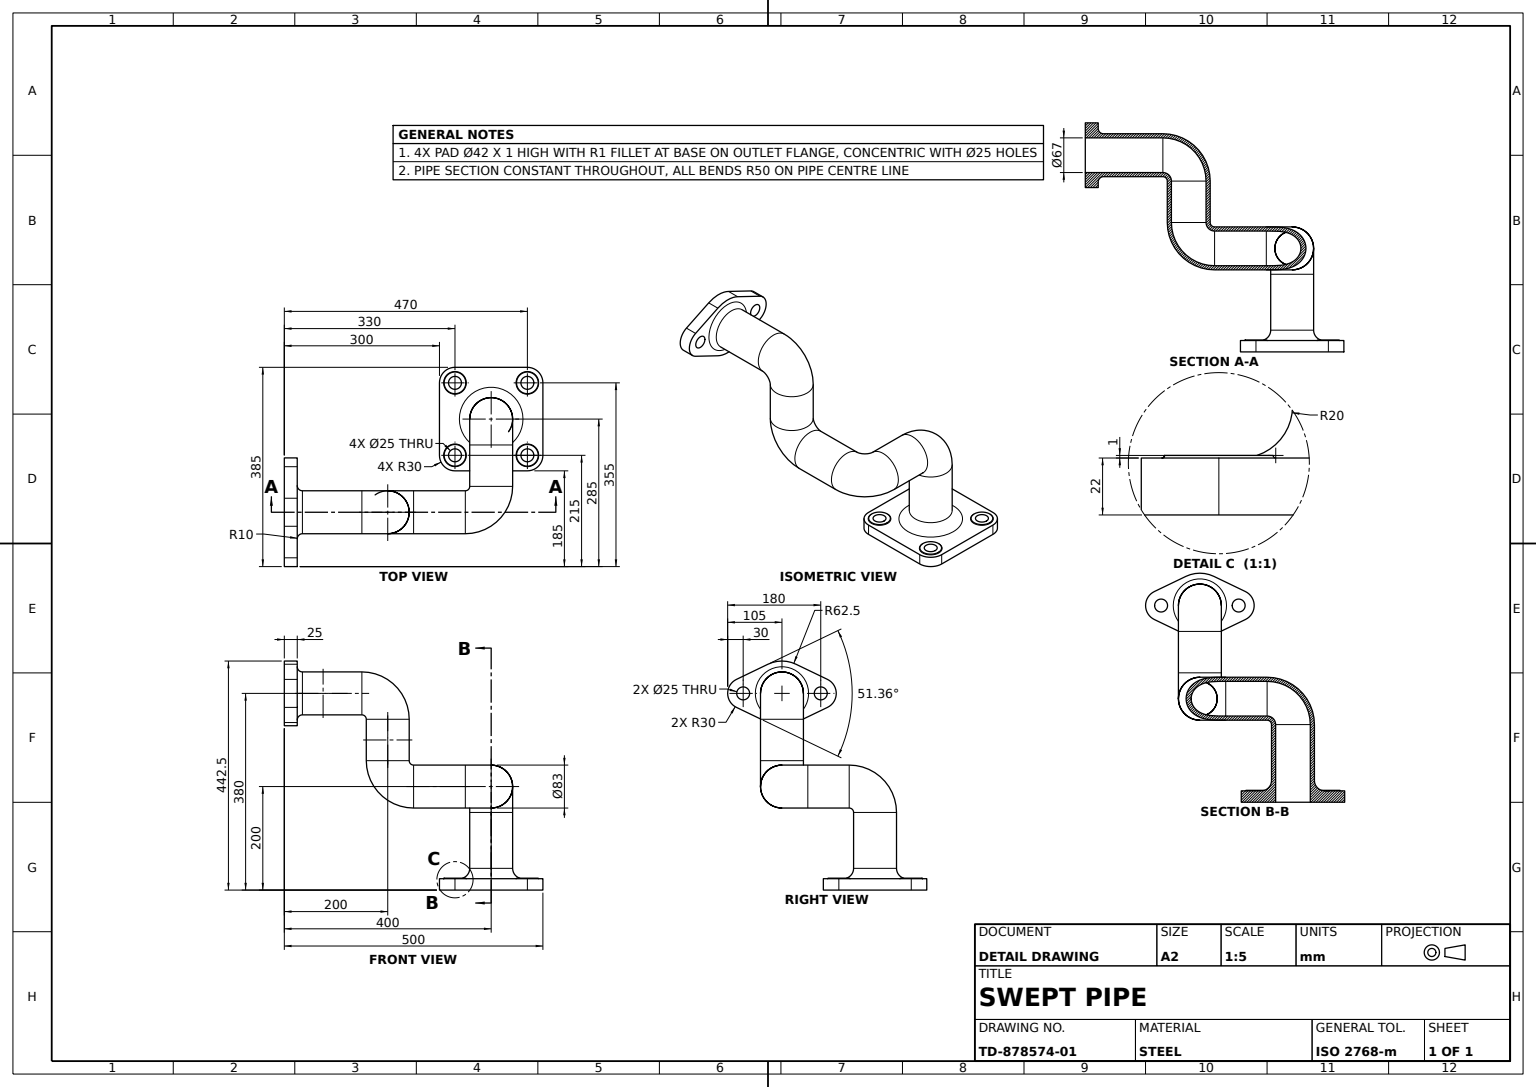
solid
v1 (70,23,49)
v2 (70,23,91)
e1 v1 v2 CIRCLE(AX(P(70,23,70),D(0,1,0),D(0,0,-1)),21)
v3 (70,22,48)
e2 v3 v1 CIRCLE(AX(P(70,23,48),D(-1,0,0),D(0,0,1)),1)
v4 (70,22,92)
e3 v4 v3 CIRCLE(AX(P(70,22,70),D(0,-1,0),D(0,0,-1)),22)
e4 v4 v2 CIRCLE(AX(P(70,23,92),D(1,0,0),D(0,0,-1)),1)
face TORUS(AX(P(70,23,70),D(0,-1,0),D(0,0,-1)),22,1) rev [-e1 -e2 -e3 e4]
v5 (100,22,-70)
v6 (100,0,-70)
e5 v5 v6 LINE
v7 (100,22,70)
e6 v5 v7 LINE
v8 (100,0,70)
e7 v7 v8 LINE
e8 v6 v8 LINE
face PLANE(AX(P(100,22,0),D(1,0,0),D(0,0,-1))) [-e5 e6 e7 -e8]
v9 (50,200,-33.5)
v10 (50,166.5,0)
e9 v9 v10 CIRCLE(AX(P(50,200,0),D(-1,0,0),D(0,-1,0)),33.5)
v11 (50,200,33.5)
e10 v10 v11 CIRCLE(AX(P(50,200,0),D(-1,0,0),D(0,-1,0)),33.5)
v12 (130,200,33.5)
e11 v11 v12 LINE
v13 (130,200,-33.5)
e12 v13 v12 CIRCLE(AX(P(130,200,0),D(-1,0,0),D(0,0,-1)),33.5)
e13 v9 v13 LINE
face CYL(AX(P(50,200,0),D(1,0,0),D(0,0,-1)),33.5) rev [e9 e10 e11 -e12 -e13]
v14 (130,200,-41.5)
v15 (130,200,41.5)
e14 v14 v15 CIRCLE(AX(P(130,200,0),D(-1,0,0),D(0,0,-1)),41.5)
v16 (221.5,200,50)
e15 v14 v16 CIRCLE(AX(P(130,200,50),D(0,-1,0),D(0,0,-1)),91.5)
v17 (138.5,200,50)
e16 v16 v17 CIRCLE(AX(P(180,200,50),D(0,0,-1),D(-1,0,0)),41.5)
e17 v15 v17 CIRCLE(AX(P(130,200,50),D(0,-1,0),D(0,0,-1)),8.5)
face TORUS(AX(P(130,200,50),D(0,-1,0),D(0,0,-1)),50,41.5) [-e14 e15 e16 -e17]
v18 (33.5,150,0)
v19 (0,150,33.5)
e18 v18 v19 CIRCLE(AX(P(0,150,0),D(0,-1,0),D(0,0,1)),33.5)
v20 (0,150,-33.5)
e19 v20 v18 CIRCLE(AX(P(0,150,0),D(0,-1,0),D(0,0,1)),33.5)
v21 (0,0,-33.5)
e20 v21 v20 LINE
v22 (0,0,33.5)
e21 v21 v22 CIRCLE(AX(P(0,0,0),D(0,-1,0),D(0,0,-1)),33.5)
e22 v22 v19 LINE
face CYL(AX(P(0,0,0),D(0,1,0),D(0,0,1)),33.5) rev [-e18 -e19 -e20 e21 e22]
v23 (221.5,380,250)
v24 (221.5,380,365)
e23 v23 v24 LINE
v25 (138.5,380,365)
e24 v24 v25 CIRCLE(AX(P(180,380,365),D(0,0,-1),D(1,0,0)),41.5)
v26 (138.5,380,250)
e25 v26 v25 LINE
v27 (180,338.5,250)
e26 v27 v26 CIRCLE(AX(P(180,380,250),D(0,0,-1),D(0,1,0)),41.5)
e27 v23 v27 CIRCLE(AX(P(180,380,250),D(0,0,-1),D(0,1,0)),41.5)
face CYL(AX(P(180,380,250),D(0,0,1),D(1,0,0)),41.5) [e23 e24 -e25 -e26 -e27]
v28 (213.5,330,200)
v29 (180,330,233.5)
e28 v28 v29 CIRCLE(AX(P(180,330,200),D(0,-1,0),D(-1,0,0)),33.5)
v30 (180,346.5,250)
e29 v29 v30 CIRCLE(AX(P(180,330,250),D(1,0,0),D(0,0,-1)),16.5)
v31 (213.5,380,250)
e30 v31 v30 CIRCLE(AX(P(180,380,250),D(0,0,-1),D(0,1,0)),33.5)
v32 (180,413.5,250)
e31 v32 v31 CIRCLE(AX(P(180,380,250),D(0,0,-1),D(0,1,0)),33.5)
v33 (180,330,166.5)
e32 v33 v32 CIRCLE(AX(P(180,330,250),D(1,0,0),D(0,0,-1)),83.5)
e33 v33 v28 CIRCLE(AX(P(180,330,200),D(0,-1,0),D(-1,0,0)),33.5)
face TORUS(AX(P(180,330,250),D(1,0,0),D(0,0,-1)),50,33.5) rev [e28 e29 -e30 -e31 -e32 e33]
v34 (-41.5,150,0)
v35 (50,241.5,0)
e34 v34 v35 CIRCLE(AX(P(50,150,0),D(0,0,-1),D(-1,0,0)),91.5)
v36 (0,150,41.5)
e35 v36 v34 CIRCLE(AX(P(0,150,0),D(0,-1,0),D(0,0,1)),41.5)
v37 (41.5,150,0)
e36 v37 v36 CIRCLE(AX(P(0,150,0),D(0,-1,0),D(0,0,1)),41.5)
v38 (50,158.5,0)
e37 v37 v38 CIRCLE(AX(P(50,150,0),D(0,0,-1),D(-1,0,0)),8.5)
v39 (50,200,41.5)
e38 v38 v39 CIRCLE(AX(P(50,200,0),D(-1,0,0),D(0,-1,0)),41.5)
e39 v39 v35 CIRCLE(AX(P(50,200,0),D(-1,0,0),D(0,-1,0)),41.5)
face TORUS(AX(P(50,150,0),D(0,0,-1),D(-1,0,0)),50,41.5) [-e34 -e35 -e36 e37 e38 e39]
v40 (92,407.037012,400)
v41 (92,352.962988,400)
e40 v40 v41 CIRCLE(AX(P(105,380,400),D(0,0,1),D(1,0,0)),30)
v42 (92,407.037012,375)
e41 v42 v40 LINE
v43 (92,352.962988,375)
e42 v42 v43 CIRCLE(AX(P(105,380,375),D(0,0,1),D(1,0,0)),30)
e43 v43 v41 LINE
face CYL(AX(P(105,380,375),D(0,0,1),D(1,0,0)),30) [-e40 -e41 e42 e43]
v44 (-70,0,82.5)
v45 (-70,0,57.5)
e44 v44 v45 CIRCLE(AX(P(-70,0,70),D(0,-1,0),D(0,0,-1)),12.5)
v46 (-70,23,57.5)
e45 v46 v45 LINE
v47 (-70,23,82.5)
e46 v46 v47 CIRCLE(AX(P(-70,23,70),D(0,1,0),D(1,0,0)),12.5)
e47 v47 v44 LINE
face CYL(AX(P(-70,22,70),D(0,-1,0),D(0,0,-1)),12.5) rev [e44 -e45 e46 e47]
v48 (146.5,380,400)
v49 (213.5,380,400)
e48 v48 v49 CIRCLE(AX(P(180,380,400),D(0,0,-1),D(-1,0,0)),33.5)
v50 (146.5,380,250)
e49 v50 v48 LINE
e50 v50 v32 CIRCLE(AX(P(180,380,250),D(0,0,-1),D(0,1,0)),33.5)
e51 v31 v49 LINE
face CYL(AX(P(180,380,250),D(0,0,1),D(1,0,0)),33.5) rev [-e48 -e49 e50 e31 e51]
v51 (70,23,-57.5)
v52 (70,0,-57.5)
e52 v51 v52 LINE
v53 (70,0,-82.5)
e53 v52 v53 CIRCLE(AX(P(70,0,-70),D(0,-1,0),D(0,0,-1)),12.5)
v54 (70,23,-82.5)
e54 v54 v53 LINE
e55 v54 v51 CIRCLE(AX(P(70,23,-70),D(0,1,0),D(-1,0,0)),12.5)
face CYL(AX(P(70,22,-70),D(0,-1,0),D(0,0,-1)),12.5) rev [e52 e53 -e54 e55]
e56 v47 v46 CIRCLE(AX(P(-70,23,70),D(0,1,0),D(1,0,0)),12.5)
v55 (-70,23,91)
v56 (-70,23,49)
e57 v55 v56 CIRCLE(AX(P(-70,23,70),D(0,1,0),D(1,0,0)),21)
e58 v56 v55 CIRCLE(AX(P(-70,23,70),D(0,1,0),D(1,0,0)),21)
face PLANE(AX(P(-70,23,70),D(0,1,0),D(1,0,0))) [-e46 -e56] [e57 e58]
v57 (268,407.037012,375)
v58 (268,407.037012,400)
e59 v57 v58 LINE
v59 (285,380,400)
e60 v59 v58 CIRCLE(AX(P(255,380,400),D(0,0,1),D(1,0,0)),30)
v60 (285,380,375)
e61 v60 v59 LINE
e62 v60 v57 CIRCLE(AX(P(255,380,375),D(0,0,1),D(1,0,0)),30)
face CYL(AX(P(255,380,375),D(0,0,1),D(1,0,0)),30) [e59 -e60 -e61 e62]
v61 (-70,23,-57.5)
v62 (-70,23,-82.5)
e63 v61 v62 CIRCLE(AX(P(-70,23,-70),D(0,1,0),D(0,0,1)),12.5)
v63 (-70,0,-82.5)
e64 v62 v63 LINE
v64 (-70,0,-57.5)
e65 v63 v64 CIRCLE(AX(P(-70,0,-70),D(0,-1,0),D(0,0,-1)),12.5)
e66 v61 v64 LINE
face CYL(AX(P(-70,22,-70),D(0,-1,0),D(0,0,-1)),12.5) rev [e63 e64 e65 -e66]
v65 (221.5,200,150)
v66 (180,158.5,150)
e67 v65 v66 CIRCLE(AX(P(180,200,150),D(0,0,-1),D(1,0,0)),41.5)
v67 (180,241.5,150)
e68 v67 v65 CIRCLE(AX(P(180,200,150),D(0,0,-1),D(1,0,0)),41.5)
v68 (180,250,158.5)
e69 v67 v68 CIRCLE(AX(P(180,250,150),D(-1,0,0),D(0,0,1)),8.5)
v69 (221.5,250,200)
e70 v68 v69 CIRCLE(AX(P(180,250,200),D(0,-1,0),D(0,0,-1)),41.5)
v70 (180,250,241.5)
e71 v69 v70 CIRCLE(AX(P(180,250,200),D(0,-1,0),D(0,0,-1)),41.5)
e72 v66 v70 CIRCLE(AX(P(180,250,150),D(-1,0,0),D(0,0,1)),91.5)
face TORUS(AX(P(180,250,150),D(-1,0,0),D(0,0,1)),50,41.5) [-e67 -e68 e69 e70 e71 -e72]
v71 (70,22,-48)
v72 (70,23,-49)
e73 v71 v72 CIRCLE(AX(P(70,23,-48),D(1,0,0),D(0,0,-1)),1)
v73 (70,22,-92)
e74 v73 v71 CIRCLE(AX(P(70,22,-70),D(0,-1,0),D(0,0,-1)),22)
v74 (70,23,-91)
e75 v73 v74 CIRCLE(AX(P(70,23,-92),D(-1,0,0),D(0,0,1)),1)
e76 v72 v74 CIRCLE(AX(P(70,23,-70),D(0,1,0),D(-1,0,0)),21)
face TORUS(AX(P(70,23,-70),D(0,-1,0),D(0,0,-1)),22,1) rev [-e73 -e74 e75 -e76]
e77 v49 v48 CIRCLE(AX(P(180,380,400),D(0,0,-1),D(-1,0,0)),33.5)
e78 v30 v50 CIRCLE(AX(P(180,380,250),D(0,0,-1),D(0,1,0)),33.5)
face CYL(AX(P(180,380,250),D(0,0,1),D(1,0,0)),33.5) rev [e49 -e77 -e51 e30 e78]
v75 (117.5,380,400)
v76 (92.5,380,400)
e79 v75 v76 CIRCLE(AX(P(105,380,400),D(0,0,1),D(1,0,0)),12.5)
v77 (92.5,380,375)
e80 v77 v76 LINE
v78 (117.5,380,375)
e81 v78 v77 CIRCLE(AX(P(105,380,375),D(0,0,1),D(1,0,0)),12.5)
e82 v78 v75 LINE
face CYL(AX(P(105,380,375),D(0,0,1),D(1,0,0)),12.5) rev [e79 -e80 -e81 e82]
e83 v15 v14 CIRCLE(AX(P(130,200,0),D(-1,0,0),D(0,0,-1)),41.5)
e84 v17 v16 CIRCLE(AX(P(180,200,50),D(0,0,-1),D(-1,0,0)),41.5)
face TORUS(AX(P(130,200,50),D(0,-1,0),D(0,0,-1)),50,41.5) [-e83 e17 e84 -e15]
v79 (138.5,200,150)
e85 v17 v79 LINE
e86 v79 v67 CIRCLE(AX(P(180,200,150),D(0,0,-1),D(1,0,0)),41.5)
e87 v16 v65 LINE
face CYL(AX(P(180,200,50),D(0,0,1),D(1,0,0)),41.5) [-e84 e85 e86 e68 -e87]
v80 (146.5,250,200)
v81 (146.5,330,200)
e88 v80 v81 LINE
v82 (180,250,166.5)
e89 v80 v82 CIRCLE(AX(P(180,250,200),D(0,-1,0),D(0,0,-1)),33.5)
v83 (213.5,250,200)
e90 v82 v83 CIRCLE(AX(P(180,250,200),D(0,-1,0),D(0,0,-1)),33.5)
e91 v83 v28 LINE
e92 v81 v33 CIRCLE(AX(P(180,330,200),D(0,-1,0),D(-1,0,0)),33.5)
face CYL(AX(P(180,250,200),D(0,1,0),D(-1,0,0)),33.5) rev [-e88 e89 e90 e91 -e33 -e92]
v84 (-70,23,-91)
v85 (-70,23,-49)
e93 v84 v85 CIRCLE(AX(P(-70,23,-70),D(0,1,0),D(0,0,1)),21)
e94 v85 v84 CIRCLE(AX(P(-70,23,-70),D(0,1,0),D(0,0,1)),21)
e95 v62 v61 CIRCLE(AX(P(-70,23,-70),D(0,1,0),D(0,0,1)),12.5)
face PLANE(AX(P(-70,23,-70),D(0,1,0),D(0,0,1))) [e93 e94] [-e63 -e95]
v86 (213.5,200,150)
v87 (180,166.5,150)
e96 v86 v87 CIRCLE(AX(P(180,200,150),D(0,0,-1),D(1,0,0)),33.5)
v88 (180,250,233.5)
e97 v87 v88 CIRCLE(AX(P(180,250,150),D(-1,0,0),D(0,0,1)),83.5)
e98 v83 v88 CIRCLE(AX(P(180,250,200),D(0,-1,0),D(0,0,-1)),33.5)
v89 (180,233.5,150)
e99 v89 v82 CIRCLE(AX(P(180,250,150),D(-1,0,0),D(0,0,1)),16.5)
e100 v89 v86 CIRCLE(AX(P(180,200,150),D(0,0,-1),D(1,0,0)),33.5)
face TORUS(AX(P(180,250,150),D(-1,0,0),D(0,0,1)),50,33.5) rev [e96 e97 -e98 -e90 -e99 e100]
v90 (-70,22,-48)
e101 v90 v85 CIRCLE(AX(P(-70,23,-48),D(1,0,0),D(0,0,-1)),1)
v91 (-70,22,-92)
e102 v91 v84 CIRCLE(AX(P(-70,23,-92),D(-1,0,0),D(0,0,1)),1)
e103 v90 v91 CIRCLE(AX(P(-70,22,-70),D(0,-1,0),D(0,0,-1)),22)
face TORUS(AX(P(-70,23,-70),D(0,-1,0),D(0,0,-1)),22,1) rev [e101 -e93 -e102 -e103]
v92 (70,23,82.5)
v93 (70,0,82.5)
e104 v92 v93 LINE
v94 (70,0,57.5)
e105 v93 v94 CIRCLE(AX(P(70,0,70),D(0,-1,0),D(0,0,-1)),12.5)
v95 (70,23,57.5)
e106 v95 v94 LINE
e107 v95 v92 CIRCLE(AX(P(70,23,70),D(0,1,0),D(0,0,-1)),12.5)
face CYL(AX(P(70,22,70),D(0,-1,0),D(0,0,-1)),12.5) rev [e104 e105 -e106 e107]
e108 v2 v1 CIRCLE(AX(P(70,23,70),D(0,1,0),D(0,0,-1)),21)
e109 v92 v95 CIRCLE(AX(P(70,23,70),D(0,1,0),D(0,0,-1)),12.5)
face PLANE(AX(P(70,23,70),D(0,1,0),D(0,0,-1))) [e108 e1] [-e109 -e107]
v96 (50,200,-41.5)
e110 v35 v96 CIRCLE(AX(P(50,200,0),D(-1,0,0),D(0,-1,0)),41.5)
e111 v39 v15 LINE
e112 v96 v14 LINE
face CYL(AX(P(50,200,0),D(1,0,0),D(0,0,-1)),41.5) [-e110 -e39 e111 e83 -e112]
v97 (-70,22,100)
v98 (-70,0,100)
e113 v97 v98 LINE
v99 (-100,22,70)
e114 v97 v99 CIRCLE(AX(P(-70,22,70),D(0,-1,0),D(0,0,-1)),30)
v100 (-100,0,70)
e115 v99 v100 LINE
e116 v98 v100 CIRCLE(AX(P(-70,0,70),D(0,-1,0),D(0,0,-1)),30)
face CYL(AX(P(-70,22,70),D(0,-1,0),D(0,0,-1)),30) [-e113 e114 e115 -e116]
e117 v64 v63 CIRCLE(AX(P(-70,0,-70),D(0,-1,0),D(0,0,-1)),12.5)
face CYL(AX(P(-70,22,-70),D(0,-1,0),D(0,0,-1)),12.5) rev [-e64 e95 e66 e117]
v101 (213.5,200,50)
e118 v101 v86 LINE
v102 (146.5,200,50)
e119 v101 v102 CIRCLE(AX(P(180,200,50),D(0,0,-1),D(-1,0,0)),33.5)
v103 (146.5,200,150)
e120 v102 v103 LINE
e121 v87 v103 CIRCLE(AX(P(180,200,150),D(0,0,-1),D(1,0,0)),33.5)
face CYL(AX(P(180,200,50),D(0,0,1),D(1,0,0)),33.5) rev [-e96 -e118 e119 e120 -e121]
e122 v76 v75 CIRCLE(AX(P(105,380,400),D(0,0,1),D(1,0,0)),12.5)
e123 v77 v78 CIRCLE(AX(P(105,380,375),D(0,0,1),D(1,0,0)),12.5)
face CYL(AX(P(105,380,375),D(0,0,1),D(1,0,0)),12.5) rev [e80 e122 -e82 -e123]
e124 v51 v54 CIRCLE(AX(P(70,23,-70),D(0,1,0),D(-1,0,0)),12.5)
e125 v53 v52 CIRCLE(AX(P(70,0,-70),D(0,-1,0),D(0,0,-1)),12.5)
face CYL(AX(P(70,22,-70),D(0,-1,0),D(0,0,-1)),12.5) rev [e124 e54 e125 -e52]
e126 v12 v102 CIRCLE(AX(P(130,200,50),D(0,-1,0),D(0,0,-1)),16.5)
e127 v13 v101 CIRCLE(AX(P(130,200,50),D(0,-1,0),D(0,0,-1)),83.5)
face TORUS(AX(P(130,200,50),D(0,-1,0),D(0,0,-1)),50,33.5) rev [e126 -e119 -e127 e12]
v104 (70,22,-100)
e128 v104 v5 CIRCLE(AX(P(70,22,-70),D(0,-1,0),D(0,0,-1)),30)
v105 (70,0,-100)
e129 v105 v6 CIRCLE(AX(P(70,0,-70),D(0,-1,0),D(0,0,-1)),30)
e130 v104 v105 LINE
face CYL(AX(P(70,22,-70),D(0,-1,0),D(0,0,-1)),30) [e128 e5 -e129 -e130]
e131 v74 v72 CIRCLE(AX(P(70,23,-70),D(0,1,0),D(-1,0,0)),21)
face PLANE(AX(P(70,23,-70),D(0,1,0),D(-1,0,0))) [-e124 -e55] [e76 e131]
v106 (138.5,250,200)
e132 v70 v106 CIRCLE(AX(P(180,250,200),D(0,-1,0),D(0,0,-1)),41.5)
v107 (221.5,330,200)
e133 v69 v107 LINE
v108 (180,330,241.5)
e134 v107 v108 CIRCLE(AX(P(180,330,200),D(0,-1,0),D(-1,0,0)),41.5)
v109 (138.5,330,200)
e135 v108 v109 CIRCLE(AX(P(180,330,200),D(0,-1,0),D(-1,0,0)),41.5)
e136 v106 v109 LINE
face CYL(AX(P(180,250,200),D(0,1,0),D(-1,0,0)),41.5) [-e132 -e71 e133 e134 e135 -e136]
v110 (-70,22,92)
v111 (-70,22,48)
e137 v110 v111 CIRCLE(AX(P(-70,22,70),D(0,-1,0),D(0,0,-1)),22)
e138 v110 v55 CIRCLE(AX(P(-70,23,92),D(1,0,0),D(0,0,-1)),1)
e139 v111 v56 CIRCLE(AX(P(-70,23,48),D(-1,0,0),D(0,0,1)),1)
face TORUS(AX(P(-70,23,70),D(0,-1,0),D(0,0,-1)),22,1) rev [-e137 e138 -e58 -e139]
e140 v96 v38 CIRCLE(AX(P(50,200,0),D(-1,0,0),D(0,-1,0)),41.5)
v112 (0,150,-41.5)
e141 v112 v37 CIRCLE(AX(P(0,150,0),D(0,-1,0),D(0,0,1)),41.5)
e142 v34 v112 CIRCLE(AX(P(0,150,0),D(0,-1,0),D(0,0,1)),41.5)
face TORUS(AX(P(50,150,0),D(0,0,-1),D(-1,0,0)),50,41.5) [e34 e110 e140 -e37 -e141 -e142]
v113 (231.5,380,375)
e143 v113 v24 CIRCLE(AX(P(231.5,380,365),D(0,-1,0),D(0,0,-1)),10)
e144 v25 v24 CIRCLE(AX(P(180,380,365),D(0,0,-1),D(1,0,0)),41.5)
v114 (128.5,380,375)
e145 v114 v25 CIRCLE(AX(P(128.5,380,365),D(0,1,0),D(-1,0,0)),10)
e146 v113 v114 CIRCLE(AX(P(180,380,375),D(0,0,1),D(1,0,0)),51.5)
face TORUS(AX(P(180,380,365),D(0,0,1),D(1,0,0)),51.5,10) rev [e143 -e144 -e145 -e146]
v115 (268,352.962988,400)
e147 v115 v59 CIRCLE(AX(P(255,380,400),D(0,0,1),D(1,0,0)),30)
v116 (268,352.962988,375)
e148 v116 v115 LINE
e149 v116 v60 CIRCLE(AX(P(255,380,375),D(0,0,1),D(1,0,0)),30)
face CYL(AX(P(255,380,375),D(0,0,1),D(1,0,0)),30) [e61 -e147 -e148 e149]
v117 (0,42,41.5)
e150 v117 v36 LINE
v118 (0,42,-41.5)
e151 v117 v118 CIRCLE(AX(P(0,42,0),D(0,1,0),D(0,0,-1)),41.5)
e152 v118 v112 LINE
face CYL(AX(P(0,0,0),D(0,1,0),D(0,0,1)),41.5) [e141 e36 -e150 e151 e152]
e153 v91 v90 CIRCLE(AX(P(-70,22,-70),D(0,-1,0),D(0,0,-1)),22)
face TORUS(AX(P(-70,23,-70),D(0,-1,0),D(0,0,-1)),22,1) rev [e102 -e94 -e101 -e153]
e154 v88 v80 CIRCLE(AX(P(180,250,200),D(0,-1,0),D(0,0,-1)),33.5)
e155 v29 v81 CIRCLE(AX(P(180,330,200),D(0,-1,0),D(-1,0,0)),33.5)
face CYL(AX(P(180,250,200),D(0,1,0),D(-1,0,0)),33.5) rev [e154 e88 -e155 -e28 -e91 e98]
v119 (-100,22,-70)
e156 v119 v99 LINE
v120 (-100,0,-70)
e157 v119 v120 LINE
e158 v120 v100 LINE
face PLANE(AX(P(-100,22,0),D(1,0,0),D(0,0,-1))) rev [-e115 -e156 e157 e158]
v121 (0,22,61.5)
e159 v121 v117 CIRCLE(AX(P(0,42,61.5),D(1,0,0),D(0,0,-1)),20)
e160 v118 v117 CIRCLE(AX(P(0,42,0),D(0,1,0),D(0,0,-1)),41.5)
v122 (0,22,-61.5)
e161 v122 v118 CIRCLE(AX(P(0,42,-61.5),D(-1,0,0),D(0,0,1)),20)
e162 v121 v122 CIRCLE(AX(P(0,22,0),D(0,-1,0),D(0,0,-1)),61.5)
face TORUS(AX(P(0,42,0),D(0,-1,0),D(0,0,-1)),61.5,20) rev [e159 -e160 -e161 -e162]
v123 (207.083333,323.672892,375)
v124 (207.083333,323.672892,400)
e163 v123 v124 LINE
e164 v123 v116 LINE
e165 v124 v115 LINE
face PLANE(AX(P(268,352.962988,375),D(0.433333333,-0.901233722,0),D(0.901233722,0.433333333,0))) [-e163 e164 e148 -e165]
v125 (207.083333,436.327108,375)
v126 (207.083333,436.327108,400)
e166 v125 v126 LINE
v127 (152.916667,436.327108,375)
e167 v125 v127 CIRCLE(AX(P(180,380,375),D(0,0,1),D(1,0,0)),62.5)
v128 (152.916667,436.327108,400)
e168 v127 v128 LINE
e169 v126 v128 CIRCLE(AX(P(180,380,400),D(0,0,1),D(1,0,0)),62.5)
face CYL(AX(P(180,380,375),D(0,0,1),D(1,0,0)),62.5) [-e166 e167 e168 -e169]
e170 v127 v42 LINE
e171 v128 v40 LINE
face PLANE(AX(P(92,407.037012,375),D(-0.433333333,0.901233722,0),D(-0.901233722,-0.433333333,0))) [e170 e41 -e171 -e168]
v129 (50,233.5,0)
e172 v11 v129 CIRCLE(AX(P(50,200,0),D(-1,0,0),D(0,-1,0)),33.5)
e173 v18 v10 CIRCLE(AX(P(50,150,0),D(0,0,-1),D(-1,0,0)),16.5)
v130 (-33.5,150,0)
e174 v19 v130 CIRCLE(AX(P(0,150,0),D(0,-1,0),D(0,0,1)),33.5)
e175 v130 v129 CIRCLE(AX(P(50,150,0),D(0,0,-1),D(-1,0,0)),83.5)
face TORUS(AX(P(50,150,0),D(0,0,-1),D(-1,0,0)),50,33.5) rev [-e172 -e10 -e173 e18 e174 e175]
v131 (152.916667,323.672892,375)
e176 v43 v131 LINE
v132 (152.916667,323.672892,400)
e177 v131 v132 LINE
e178 v41 v132 LINE
face PLANE(AX(P(92,352.962988,375),D(-0.433333333,-0.901233722,0),D(0.901233722,-0.433333333,0))) [e176 e177 -e178 -e43]
v133 (267.5,380,375)
v134 (242.5,380,375)
e179 v133 v134 CIRCLE(AX(P(255,380,375),D(0,0,1),D(1,0,0)),12.5)
v135 (267.5,380,400)
e180 v133 v135 LINE
v136 (242.5,380,400)
e181 v135 v136 CIRCLE(AX(P(255,380,400),D(0,0,1),D(1,0,0)),12.5)
e182 v134 v136 LINE
face CYL(AX(P(255,380,375),D(0,0,1),D(1,0,0)),12.5) rev [-e179 e180 e181 -e182]
e183 v45 v44 CIRCLE(AX(P(-70,0,70),D(0,-1,0),D(0,0,-1)),12.5)
face CYL(AX(P(-70,22,70),D(0,-1,0),D(0,0,-1)),12.5) rev [e56 e45 e183 -e47]
e184 v71 v73 CIRCLE(AX(P(70,22,-70),D(0,-1,0),D(0,0,-1)),22)
face TORUS(AX(P(70,23,-70),D(0,-1,0),D(0,0,-1)),22,1) rev [-e184 e73 -e131 -e75]
v137 (180,330,158.5)
e185 v109 v137 CIRCLE(AX(P(180,330,200),D(0,-1,0),D(-1,0,0)),41.5)
e186 v137 v107 CIRCLE(AX(P(180,330,200),D(0,-1,0),D(-1,0,0)),41.5)
e187 v106 v68 CIRCLE(AX(P(180,250,200),D(0,-1,0),D(0,0,-1)),41.5)
face CYL(AX(P(180,250,200),D(0,1,0),D(-1,0,0)),41.5) [e136 e185 e186 -e133 -e70 -e187]
v138 (180,421.5,250)
e188 v138 v23 CIRCLE(AX(P(180,380,250),D(0,0,-1),D(0,1,0)),41.5)
e189 v108 v27 CIRCLE(AX(P(180,330,250),D(1,0,0),D(0,0,-1)),8.5)
e190 v137 v138 CIRCLE(AX(P(180,330,250),D(1,0,0),D(0,0,-1)),91.5)
face TORUS(AX(P(180,330,250),D(1,0,0),D(0,0,-1)),50,41.5) [e188 e27 -e189 -e134 -e186 e190]
e191 v103 v89 CIRCLE(AX(P(180,200,150),D(0,0,-1),D(1,0,0)),33.5)
face TORUS(AX(P(180,250,150),D(-1,0,0),D(0,0,1)),50,33.5) rev [-e89 -e154 -e97 e121 e191 e99]
e192 v114 v113 CIRCLE(AX(P(180,380,375),D(0,0,1),D(1,0,0)),51.5)
e193 v131 v123 CIRCLE(AX(P(180,380,375),D(0,0,1),D(1,0,0)),62.5)
e194 v57 v125 LINE
e195 v134 v133 CIRCLE(AX(P(255,380,375),D(0,0,1),D(1,0,0)),12.5)
face PLANE(AX(P(105,380,375),D(0,0,1),D(1,0,0))) rev [e146 e192] [-e62 -e149 -e164 -e193 -e176 -e42 -e170 -e167 -e194] [e195 e179] [e123 e81]
e196 v58 v126 LINE
face PLANE(AX(P(268,407.037012,375),D(0.433333333,0.901233722,0),D(-0.901233722,0.433333333,0))) [-e196 -e59 e194 e166]
face CYL(AX(P(0,0,0),D(0,1,0),D(0,0,1)),41.5) [-e152 e160 e150 e35 e142]
v139 (-70,0,-100)
e197 v105 v139 LINE
v140 (-70,22,-100)
e198 v140 v139 LINE
e199 v104 v140 LINE
face PLANE(AX(P(0,22,-100),D(0,0,1),D(1,0,0))) rev [e130 e197 -e198 -e199]
e200 v94 v93 CIRCLE(AX(P(70,0,70),D(0,-1,0),D(0,0,-1)),12.5)
v141 (70,0,100)
e201 v8 v141 CIRCLE(AX(P(70,0,70),D(0,-1,0),D(0,0,-1)),30)
e202 v141 v98 LINE
e203 v139 v120 CIRCLE(AX(P(-70,0,-70),D(0,1,0),D(0,0,-1)),30)
e204 v22 v21 CIRCLE(AX(P(0,0,0),D(0,-1,0),D(0,0,-1)),33.5)
face PLANE(AX(P(0,0,0),D(0,-1,0),D(0,0,1))) [-e53 -e125] [-e200 -e105] [-e117 -e65] [-e183 -e44] [e201 e202 e116 -e158 -e203 -e197 e129 e8] [-e21 -e204]
face TORUS(AX(P(180,330,250),D(1,0,0),D(0,0,-1)),50,33.5) rev [-e29 e155 e92 e32 -e50 -e78]
e205 v66 v79 CIRCLE(AX(P(180,200,150),D(0,0,-1),D(1,0,0)),41.5)
face CYL(AX(P(180,200,50),D(0,0,1),D(1,0,0)),41.5) [e87 e67 e205 -e85 -e16]
v142 (70,22,100)
e206 v142 v141 LINE
e207 v7 v142 CIRCLE(AX(P(70,22,70),D(0,-1,0),D(0,0,-1)),30)
face CYL(AX(P(70,22,70),D(0,-1,0),D(0,0,-1)),30) [e206 -e201 -e7 e207]
e208 v129 v9 CIRCLE(AX(P(50,200,0),D(-1,0,0),D(0,-1,0)),33.5)
e209 v130 v20 CIRCLE(AX(P(0,150,0),D(0,-1,0),D(0,0,1)),33.5)
face TORUS(AX(P(50,150,0),D(0,0,-1),D(-1,0,0)),50,33.5) rev [-e9 -e208 -e175 e209 e19 e173]
e210 v111 v110 CIRCLE(AX(P(-70,22,70),D(0,-1,0),D(0,0,-1)),22)
e211 v142 v97 LINE
e212 v140 v119 CIRCLE(AX(P(-70,22,-70),D(0,1,0),D(0,0,-1)),30)
e213 v122 v121 CIRCLE(AX(P(0,22,0),D(0,-1,0),D(0,0,-1)),61.5)
e214 v3 v4 CIRCLE(AX(P(70,22,70),D(0,-1,0),D(0,0,-1)),22)
face PLANE(AX(P(0,22,0),D(0,-1,0),D(0,0,-1))) rev [e210 e137] [-e114 -e211 -e207 -e6 -e128 e199 e212 e156] [e213 e162] [e3 e214] [e74 e184] [e153 e103]
e215 v102 v101 CIRCLE(AX(P(180,200,50),D(0,0,-1),D(-1,0,0)),33.5)
face CYL(AX(P(180,200,50),D(0,0,1),D(1,0,0)),33.5) rev [e215 e118 -e100 -e191 -e120]
e216 v132 v124 CIRCLE(AX(P(180,380,400),D(0,0,1),D(1,0,0)),62.5)
face CYL(AX(P(180,380,375),D(0,0,1),D(1,0,0)),62.5) [-e216 -e177 e193 e163]
face TORUS(AX(P(70,23,70),D(0,-1,0),D(0,0,-1)),22,1) rev [-e4 -e214 e2 -e108]
face TORUS(AX(P(180,380,365),D(0,0,1),D(1,0,0)),51.5,10) rev [-e24 -e143 -e192 e145]
e217 v26 v138 CIRCLE(AX(P(180,380,250),D(0,0,-1),D(0,1,0)),41.5)
face CYL(AX(P(180,380,250),D(0,0,1),D(1,0,0)),41.5) [e25 e144 -e23 -e188 -e217]
face CYL(AX(P(70,22,70),D(0,-1,0),D(0,0,-1)),12.5) rev [e106 e200 -e104 e109]
face PLANE(AX(P(0,22,100),D(0,0,1),D(1,0,0))) [e113 -e202 -e206 e211]
e218 v12 v13 CIRCLE(AX(P(130,200,0),D(-1,0,0),D(0,0,-1)),33.5)
face CYL(AX(P(50,200,0),D(1,0,0),D(0,0,-1)),33.5) rev [-e11 e172 e208 e13 -e218]
face TORUS(AX(P(180,330,250),D(1,0,0),D(0,0,-1)),50,41.5) [e217 -e190 -e185 -e135 e189 e26]
face CYL(AX(P(-70,22,-70),D(0,-1,0),D(0,0,-1)),30) [e203 -e157 -e212 e198]
face TORUS(AX(P(0,42,0),D(0,-1,0),D(0,0,-1)),61.5,20) rev [e161 -e151 -e159 -e213]
face TORUS(AX(P(130,200,50),D(0,-1,0),D(0,0,-1)),50,33.5) rev [e218 e127 -e215 -e126]
face TORUS(AX(P(-70,23,70),D(0,-1,0),D(0,0,-1)),22,1) rev [e139 -e57 -e138 -e210]
face CYL(AX(P(0,0,0),D(0,1,0),D(0,0,1)),33.5) rev [e20 -e209 -e174 -e22 e204]
e219 v136 v135 CIRCLE(AX(P(255,380,400),D(0,0,1),D(1,0,0)),12.5)
face CYL(AX(P(255,380,375),D(0,0,1),D(1,0,0)),12.5) rev [e182 e219 -e180 -e195]
face CYL(AX(P(50,200,0),D(1,0,0),D(0,0,-1)),41.5) [e112 e14 -e111 -e38 -e140]
face PLANE(AX(P(180,380,400),D(0,0,-1),D(-1,0,0))) rev [e216 e165 e147 e60 e196 e169 e171 e40 e178] [-e79 -e122] [e77 e48] [-e181 -e219]
face TORUS(AX(P(180,250,150),D(-1,0,0),D(0,0,1)),50,41.5) [-e69 -e86 -e205 e72 e132 e187]
